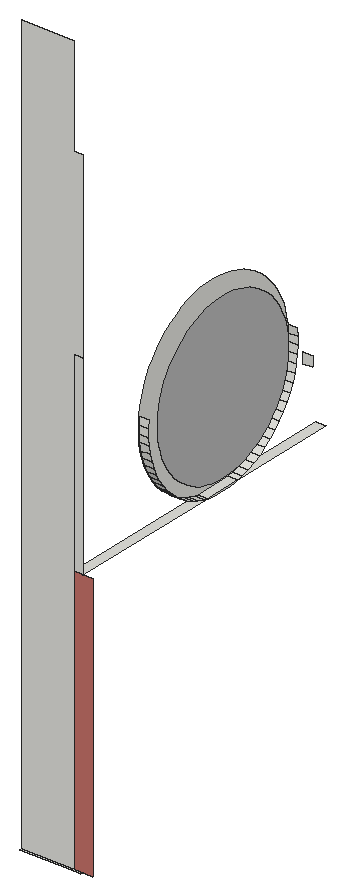
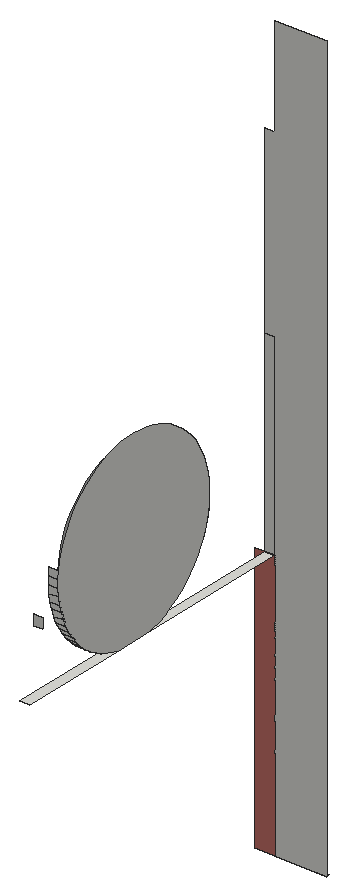
# SketchUp Ruby script. Lengths in inches.
U = 1.inch
M = Sketchup.active_model
def pt(a) = Geom::Point3d.new(a.map { |v| v * U })
def face(e, loops, mat)
  f = e.add_face(loops[0].map { |a| pt(a) })
  loops[1..].each { |l| e.add_face(l.map { |a| pt(a) }).erase! }
  f.material = f.back_material = mat if mat
  f
end
# faces: each face lists its corners as indices into pts; further lists are holes
def faces(e, pts, list, mat = nil) = list.each { |f| face(e, (f[0].is_a?(Array) ? f : [f]).map { |l| l.map { |i| pts[i] } }, mat) }
# xy, xz, yz: faces in a plane at the given z, y or x. An outline is a flat list of corners, or four numbers for a rectangle; further outlines are holes
def ring(l) = l.size == 4 ? [[l[0], l[1]], [l[2], l[1]], [l[2], l[3]], [l[0], l[3]]] : l.each_slice(2).to_a
def flat(e, list, mat, &to3) = list.each { |f| face(e, (f[0].is_a?(Array) ? f : [f]).map { |l| ring(l).map { |u, v| to3.(u, v) } }, mat) }
def xy(e, z, list, mat = nil) = flat(e, list, mat) { |x, y| [x, y, z] }
def xz(e, y, list, mat = nil) = flat(e, list, mat) { |x, z| [x, y, z] }
def yz(e, x, list, mat = nil) = flat(e, list, mat) { |y, z| [x, y, z] }
def lines(e, pts, list) = list.each { |a, b| e.add_line(pt(pts[a]), pt(pts[b])) }
# prism: a flat outline (further loops are holes) pulled along v
def prism(e, loops, v, mat = nil)
  f = face(e, loops, mat); d = Geom::Vector3d.new(v.map { |x| x * U })
  f.pushpull(f.normal.samedirection?(d) ? d.length : -d.length)
end
def box(e, o, s, mat = nil) = prism(e, [[o, [o[0] + s[0], o[1], o[2]], [o[0] + s[0], o[1] + s[1], o[2]], [o[0], o[1] + s[1], o[2]]]], [0, 0, s[2]], mat)
def at(x, y, z, deg = 0) = Geom::Transformation.translation(pt([x, y, z])) * Geom::Transformation.rotation(ORIGIN, Z_AXIS, deg.degrees)
def axes(o, x, y, z) = Geom::Transformation.new([*x, 0, *y, 0, *z, 0, *pt(o).to_a, 1])
def part(name) = M.definitions.add(name)
# library, detail: a bought-in or finely detailed component or shape, given as its bounding box
def library(name, o, s) = part(name).tap { |d| box(d.entities, o, s) }
def detail(e, o, s) = box(e.add_group.entities, o, s)
def put(e, d, t, mat = nil) = e.add_instance(d, t).tap { |i| i.material = mat if mat }
def group(e, t, mat = nil) = e.add_group.tap { |g| g.transformation = t; g.material = mat if mat }.entities
root = M.entities
M.materials.add("[Mirror 01]").color = [185, 185, 185]
M.materials.add("[Wood Floor Dark]").color = [198, 114, 106]
xy(root,0,[[0,0,9,0.4375],[9,0,10.6875,0.4375]])
xy(root,46.5,[[9,0.4375,10.6875,27.54],[9,27.54,10.6875,34.125],[9,34.125,10.6875,53.23]])
xz(root,0.4375,[[0,0,9,0,9,80.35,10.6875,80.35,10.6875,112.04,9,112.04,9,129.25,0,129.25],[9,46.5,10.6875,80.35]])
xz(root,0.4375,[[9,0,12.375,46.5]],"[Wood Floor Dark]")
xz(root,14.55,[[9,61.68,10.6875,63.06]])
xz(root,50.33,[[9,56.96,10.6875,58.74]])
yz(root,9,[[27.54,46.5,34.125,46.5,35.01,46.69,36.33,47.11,37.61,47.625,38.84,48.25,40.02,48.99,41.125,49.8125,42.16,50.73,43.11,51.73,43.98,52.8125,44.75,53.96,45.42,55.17,45.98,56.4375,46.43,57.74,46.78,59.08,47,60.45,47.12,61.83,47.11,63.21,46.99,64.59,46.75,65.95,46.39,67.29,45.93,68.59,45.35,69.85,44.67,71.05,43.89,72.19,43.02,73.27,42.06,74.26,41.01,75.17,39.9,75.99,38.72,76.71,37.48,77.32,36.19,77.83,34.87,78.23,33.51,78.52,32.14,78.6875,30.76,78.74,29.38,78.68,28.01,78.49,26.66,78.2,25.34,77.79,24.05,77.26,22.82,76.64,21.65,75.91,20.54,75.08,19.5,74.16,18.55,73.16,17.6875,72.08,16.92,70.93,16.25,69.72,15.68,68.45,15.23,67.15,14.89,65.81,14.66,64.44,14.55,63.06,14.55,61.68,14.68,60.3,14.92,58.94,15.27,57.6,15.74,56.3,16.3125,55.04,16.99,53.84,17.77,52.7,18.65,51.625,19.61,50.63,20.65,49.72,21.77,48.9,22.95,48.18,24.1875,47.57,25.47,47.06,26.8,46.66]])
yz(root,10.6875,[[30.9,46.15,32.29,46.22,33.66,46.4,34.125,46.5,27.54,46.5,28.15,46.37,29.52,46.2]])
yz(root,10.6875,[[30.9,48.2,32.1,48.25,33.3,48.41,34.48,48.67,35.64,49.03,36.76,49.49,37.84,50.04,38.86,50.67,39.83,51.4,40.74,52.2,41.57,53.08,42.33,54.02,43,55.03,43.58,56.09,44.08,57.19,44.48,58.33,44.78,59.51,44.97,60.7,45.07,61.9,45.07,63.11,44.96,64.32,44.75,65.51,44.4375,66.68,44.03,67.82,43.53,68.92,42.93,69.97,42.25,70.97,41.49,71.91,40.65,72.78,39.73,73.57,38.76,74.29,37.73,74.92,36.64,75.46,35.52,75.9,34.36,76.25,33.18,76.5,31.98,76.65,30.77,76.7,29.56,76.64,28.36,76.48,27.18,76.22,26.03,75.86,24.9,75.4,23.83,74.86,22.8,74.22,21.83,73.49,20.93,72.69,20.09,71.8125,19.34,70.87,18.66,69.86,18.08,68.8,17.59,67.7,17.1875,66.56,16.89,65.39,16.6875,64.19,16.59,62.99,16.6,61.78,16.71,60.57,16.92,59.38,17.23,58.21,17.63,57.07,18.14,55.97,18.73,54.92,19.41,53.92,20.18,52.98,21.02,52.11,21.93,51.32,22.9,50.6,23.9375,49.97,25.02,49.43,26.14,48.99,27.3,48.64,28.49,48.39,29.6875,48.24]],"[Mirror 01]")
p = [[10.6875,26.8,46.66],[10.6875,27.54,46.5],[9,27.54,46.5],[9,26.8,46.66],[10.6875,34.125,46.5],[10.6875,35.01,46.69],
  [9,35.01,46.69],[9,34.125,46.5],[10.6875,25.47,47.06],[9,25.47,47.06],[10.6875,36.33,47.11],[9,36.33,47.11],
  [10.6875,24.1875,47.57],[9,24.1875,47.57],[10.6875,37.61,47.625],[9,37.61,47.625],[10.6875,22.95,48.18],[9,22.95,48.18],
  [10.6875,38.84,48.25],[9,38.84,48.25],[10.6875,21.77,48.9],[9,21.77,48.9],[10.6875,40.02,48.99],[9,40.02,48.99],
  [10.6875,20.65,49.72],[9,20.65,49.72],[10.6875,41.125,49.8125],[9,41.125,49.8125],[10.6875,19.61,50.63],[9,19.61,50.63],
  [10.6875,42.16,50.73],[9,42.16,50.73],[10.6875,18.65,51.625],[9,18.65,51.625],[10.6875,43.11,51.73],[9,43.11,51.73],
  [10.6875,17.77,52.7],[9,17.77,52.7],[10.6875,43.98,52.8125],[9,43.98,52.8125],[10.6875,16.99,53.84],[9,16.99,53.84],
  [10.6875,44.75,53.96],[9,44.75,53.96],[10.6875,16.3125,55.04],[9,16.3125,55.04],[10.6875,45.42,55.17],[9,45.42,55.17],
  [10.6875,15.74,56.3],[9,15.74,56.3],[10.6875,45.98,56.4375],[9,45.98,56.4375],[10.6875,15.27,57.6],[9,15.27,57.6],
  [10.6875,46.43,57.74],[9,46.43,57.74],[10.6875,14.92,58.94],[9,14.92,58.94],[10.6875,46.78,59.08],[9,46.78,59.08],
  [10.6875,14.68,60.3],[9,14.68,60.3],[10.6875,47,60.45],[9,47,60.45],[10.6875,14.55,61.68],[9,14.55,61.68],
  [10.6875,47.12,61.83],[9,47.12,61.83],[10.6875,47.11,63.21],[9,47.11,63.21],[10.6875,14.66,64.44],[10.6875,14.55,63.06],
  [9,14.55,63.06],[9,14.66,64.44],[10.6875,46.99,64.59],[9,46.99,64.59]]
faces(root,p,[[0,1,2,3],[4,5,6,7],[8,0,3,9],[5,10,11,6],[12,8,9,13],[10,14,15,11],[16,12,13,17],[14,18,19,15],
  [20,16,17,21],[18,22,23,19],[24,20,21,25],[22,26,27,23],[28,24,25,29],[26,30,31,27],[32,28,29,33],[30,34,35,31],
  [36,32,33,37],[34,38,39,35],[40,36,37,41],[38,42,43,39],[44,40,41,45],[42,46,47,43],[48,44,45,49],[46,50,51,47],
  [52,48,49,53],[50,54,55,51],[56,52,53,57],[54,58,59,55],[60,56,57,61],[58,62,63,59],[64,60,61,65],[62,66,67,63],
  [66,68,69,67],[70,71,72,73],[68,74,75,69]])
